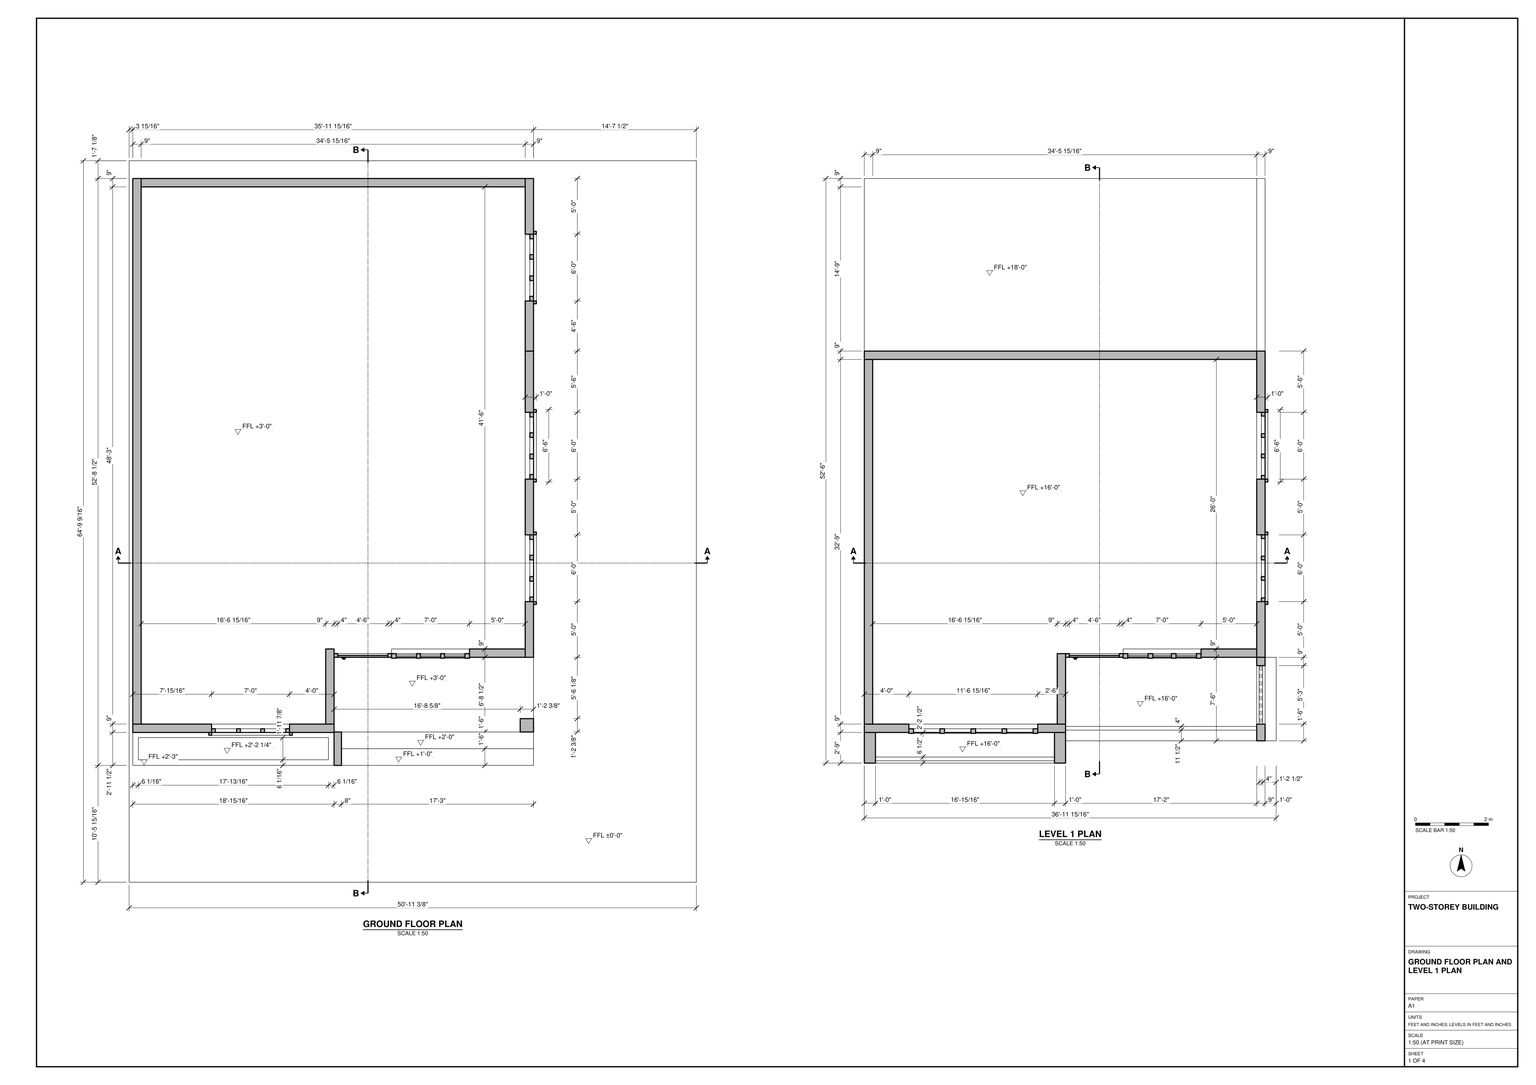
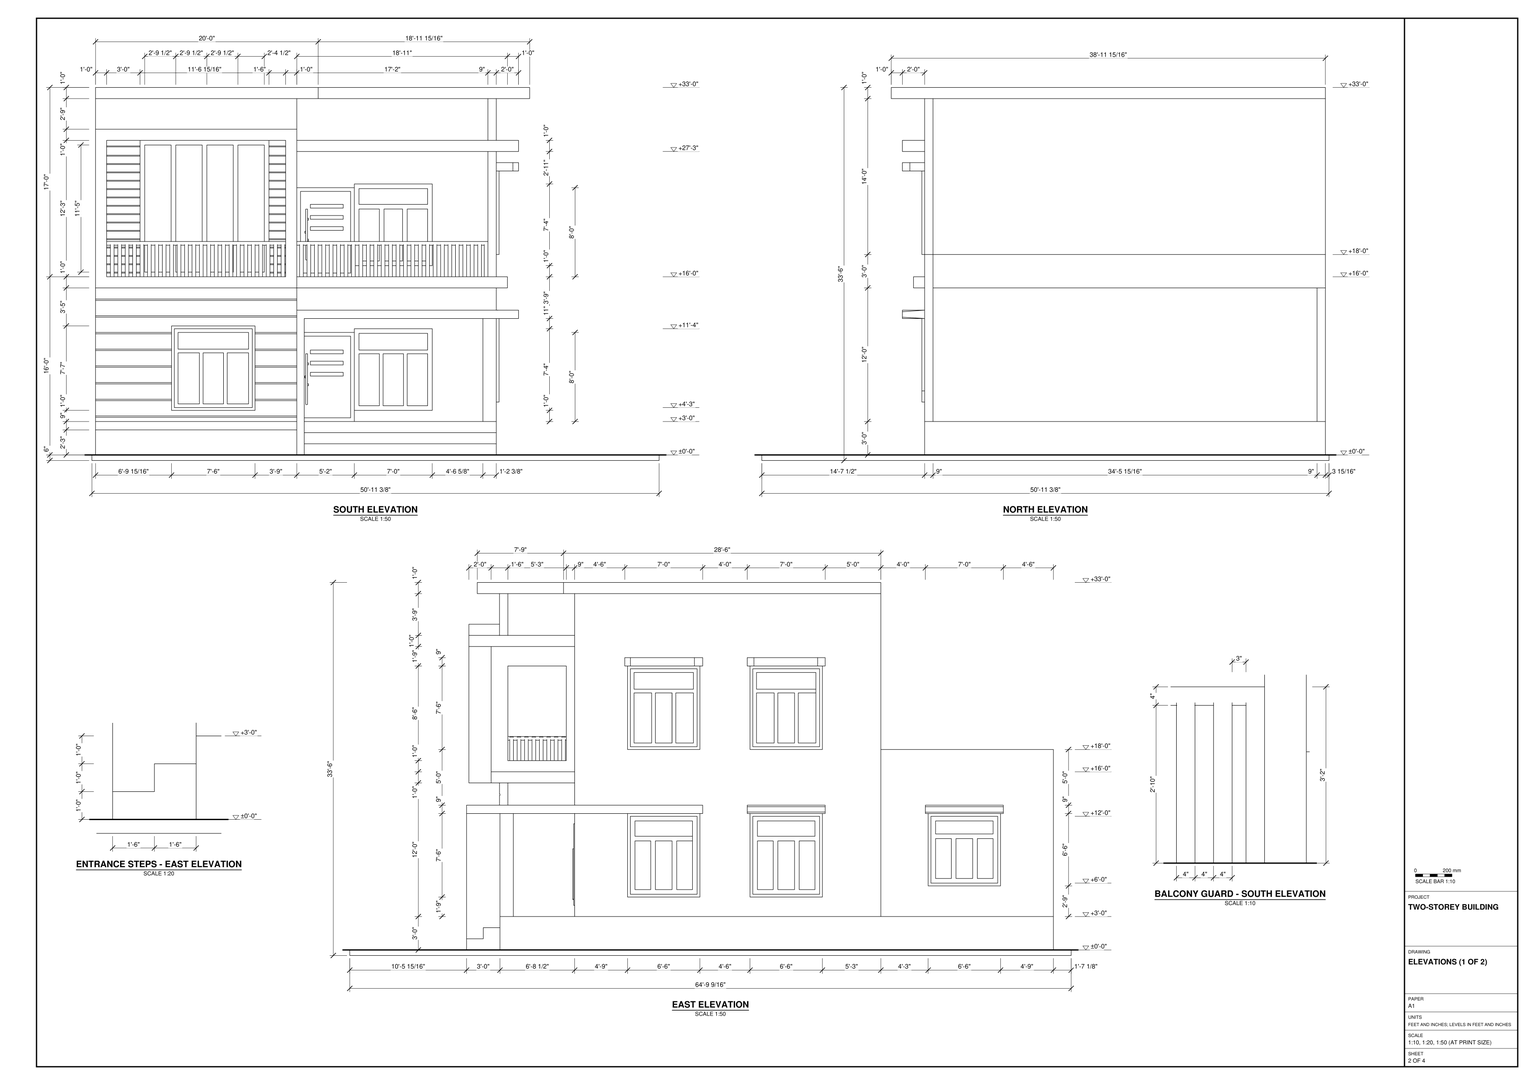
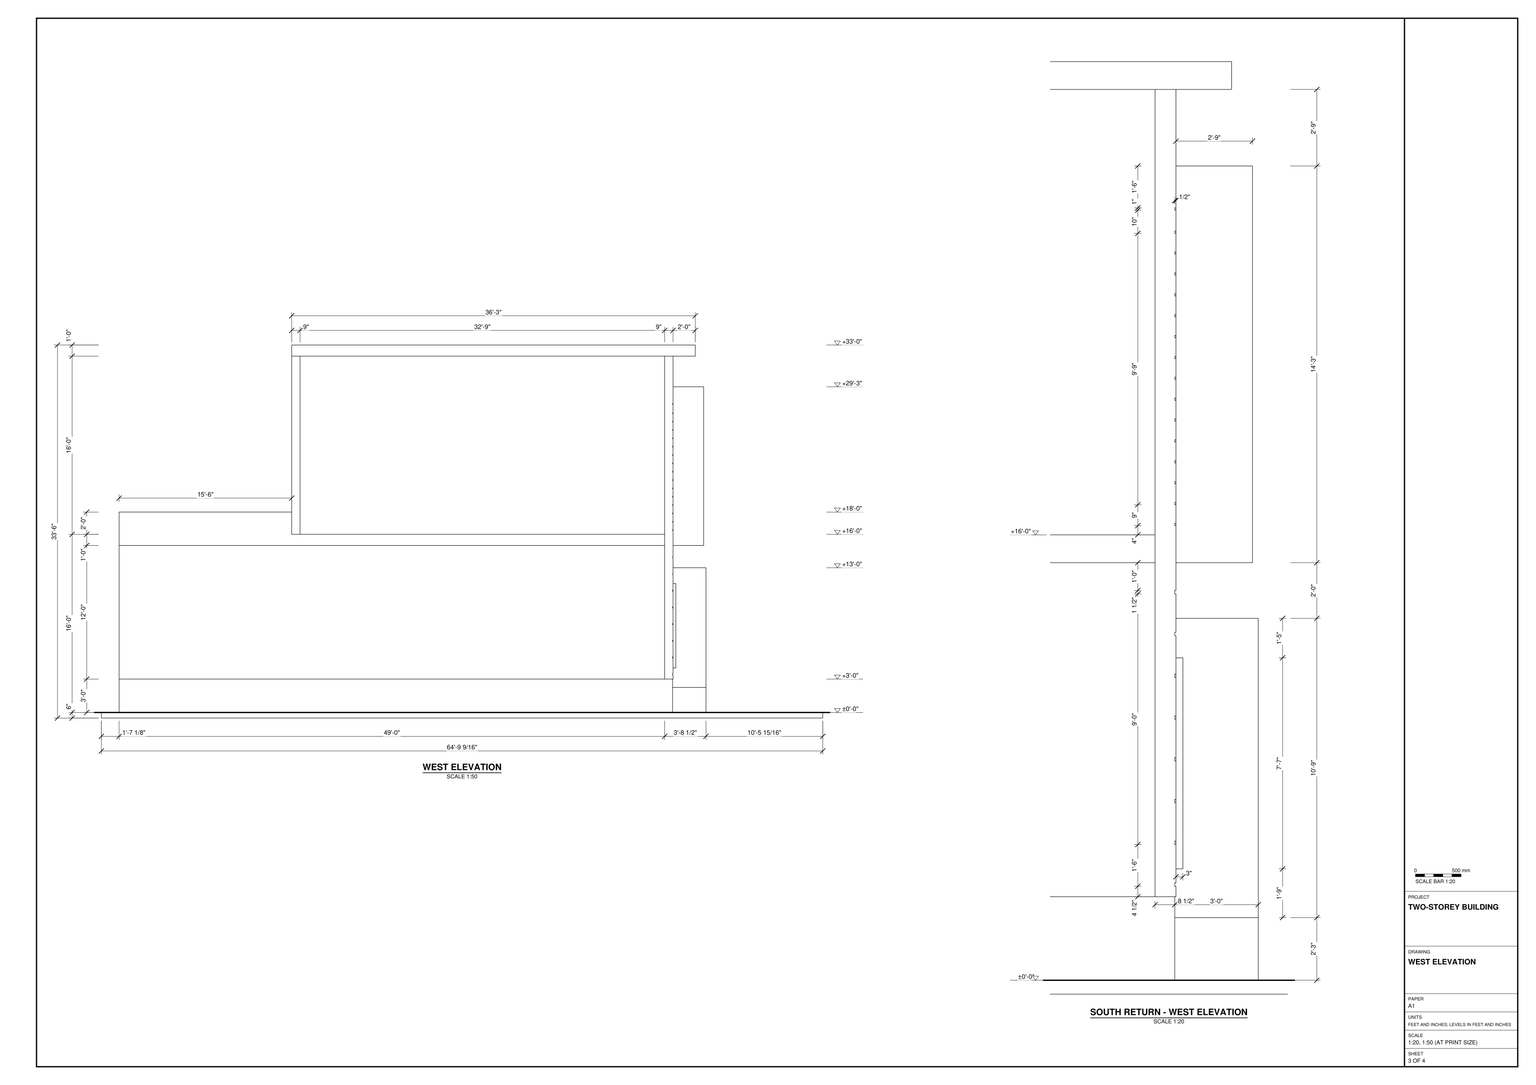
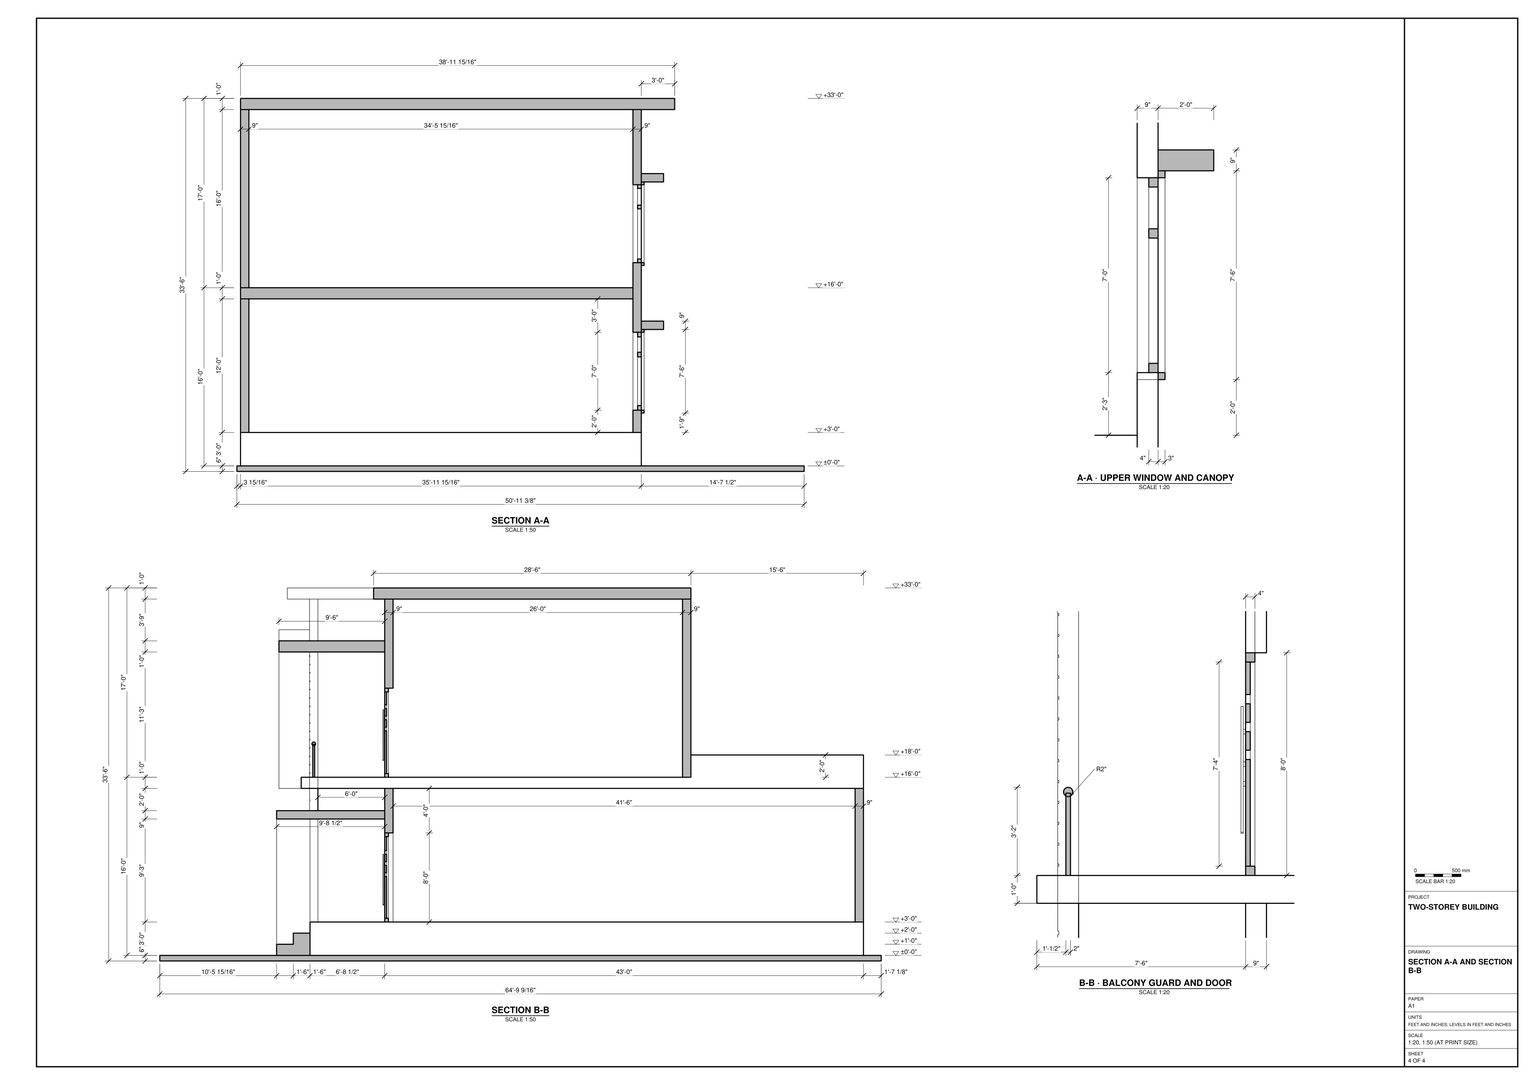
Build the two-storey building and its rectangular site base in SketchUp using task_files/diagram_01.pdf. Work in feet and inches. With north at the top of the plan, make the complete model 50'-11 3/8" wide, 64'-9 9/16" deep and 33'-6" high, including the base. Use ±0'-0" as the ground datum and +16'-0" as the upper storey level. Raise the ground floor and entrance landing to +3'-0" above the datum.

Set out the perimeter walls at the thicknesses drawn, retaining the recess at the south entrance. Model the floor slabs, the lower rear roof with its raised edge, and the flat overhanging roof above the shorter upper storey. Build the entrance steps, the porch supports and the upper balcony with its vertical guard bars. Use the south elevation to place the doors and divided windows, the horizontal bands on the projecting bay and the canopies over the recessed bay. Match the east window openings and their projecting heads to the elevation; keep the north and west walls unpierced.

Keep walls, slabs and roofs in separate groups or components. Group each furniture or joinery piece separately where shown, and use components for repeated parts. Any decor or loose items shown may be suitable library components. Save one SketchUp model as output_files/two_storey_building_with_stepped_entrance_and_balcony.skp.

# SketchUp Ruby script. Lengths in inches.
U = 1.inch
M = Sketchup.active_model
def pt(a) = Geom::Point3d.new(a.map { |v| v * U })
def face(e, loops, mat)
  f = e.add_face(loops[0].map { |a| pt(a) })
  loops[1..].each { |l| e.add_face(l.map { |a| pt(a) }).erase! }
  f.material = f.back_material = mat if mat
  f
end
# faces: each face lists its corners as indices into pts; further lists are holes
def faces(e, pts, list, mat = nil) = list.each { |f| face(e, (f[0].is_a?(Array) ? f : [f]).map { |l| l.map { |i| pts[i] } }, mat) }
# xy, xz, yz: faces in a plane at the given z, y or x. An outline is a flat list of corners, or four numbers for a rectangle; further outlines are holes
def ring(l) = l.size == 4 ? [[l[0], l[1]], [l[2], l[1]], [l[2], l[3]], [l[0], l[3]]] : l.each_slice(2).to_a
def flat(e, list, mat, &to3) = list.each { |f| face(e, (f[0].is_a?(Array) ? f : [f]).map { |l| ring(l).map { |u, v| to3.(u, v) } }, mat) }
def xy(e, z, list, mat = nil) = flat(e, list, mat) { |x, y| [x, y, z] }
def xz(e, y, list, mat = nil) = flat(e, list, mat) { |x, z| [x, y, z] }
def yz(e, x, list, mat = nil) = flat(e, list, mat) { |y, z| [x, y, z] }
def lines(e, pts, list) = list.each { |a, b| e.add_line(pt(pts[a]), pt(pts[b])) }
# prism: a flat outline (further loops are holes) pulled along v
def prism(e, loops, v, mat = nil)
  f = face(e, loops, mat); d = Geom::Vector3d.new(v.map { |x| x * U })
  f.pushpull(f.normal.samedirection?(d) ? d.length : -d.length)
end
def box(e, o, s, mat = nil) = prism(e, [[o, [o[0] + s[0], o[1], o[2]], [o[0] + s[0], o[1] + s[1], o[2]], [o[0], o[1] + s[1], o[2]]]], [0, 0, s[2]], mat)
def at(x, y, z, deg = 0) = Geom::Transformation.translation(pt([x, y, z])) * Geom::Transformation.rotation(ORIGIN, Z_AXIS, deg.degrees)
def axes(o, x, y, z) = Geom::Transformation.new([*x, 0, *y, 0, *z, 0, *pt(o).to_a, 1])
def part(name) = M.definitions.add(name)
# library, detail: a bought-in or finely detailed component or shape, given as its bounding box
def library(name, o, s) = part(name).tap { |d| box(d.entities, o, s) }
def detail(e, o, s) = box(e.add_group.entities, o, s)
def put(e, d, t, mat = nil) = e.add_instance(d, t).tap { |i| i.material = mat if mat }
def group(e, t, mat = nil) = e.add_group.tap { |g| g.transformation = t; g.material = mat if mat }.entities
root = M.entities
M.materials.add("[Color D06]").color = [142, 107, 0]
M.materials.add("[Color M02]").color = [198, 198, 198]
M.materials.add("[Color M04]").color = [142, 142, 142]
M.materials.add("[Color M05]").color = [114, 114, 114]
M.materials.add("[Color M06]").color = [86, 86, 86]
M.materials.add("[Color M09]").color = [0, 0, 0]
M.materials.add("[Grass Dark Green]").color = [106, 157, 55]
M.materials.add("[Pavers with Grass Brick]").color = [187, 192, 176]
M.materials.add("[Translucent Glass Gray]").color = [128, 128, 128]
M.materials["[Translucent Glass Gray]"].alpha = 0.5
M.materials.add("[Wood Veneer 01]").color = [109, 63, 33]
M.materials.add("[Wood Veneer 01]1").color = [73, 43, 22]
c1 = part("Group\#26")
box(c1.entities,[0,0,0],[3,1,2])
c2 = part("Group\#27")
box(c2.entities,[-1,0,0],[3,1,2])
c3 = part("Group\#28")
box(c3.entities,[0,0,0],[3,1,2])
c4 = part("Group\#29")
prism(c4.entities,[[[0,1,30.5],[2,1,30.5],[2,1,-23.76],[2,1,-23.82],[1.98,1,-23.88],[1.96,1,-23.94],[1.93,1,-24],[1.9,1,-24.06],[1.86,1,-24.11],[1.81,1,-24.15],[1.75,1,-24.18],[1.69,1,-24.21],[1.63,1,-24.23],[1.57,1,-24.25],[1.51,1,-24.25],[0.52,1,-24.25],[0.45,1,-24.25],[0.38,1,-24.23],[0.32,1,-24.21],[0.26,1,-24.18],[0.2,1,-24.14],[0.15,1,-24.1],[0.11,1,-24.05],[0.07,1,-23.99],[0.04,1,-23.93],[0.02,1,-23.87],[0,1,-23.8],[0,1,-23.73]]],[0,-1,0])
c5 = part("Group\#40")
prism(c5.entities,[[[74,0.51,0.02],[74,0.6875,0],[74,0.87,0.02],[74,1.03,0.09],[74,1.17,0.2],[74,1.28,0.34],[74,1.35,0.51],[74,1.375,0.6875],[74,1.35,0.87],[74,1.28,1.03],[74,1.17,1.17],[74,1.03,1.28],[74,0.87,1.35],[74,0.6875,1.375],[74,0.51,1.35],[74,0.34,1.28],[74,0.2,1.17],[74,0.09,1.03],[74,0.02,0.87],[74,0,0.6875],[74,0.02,0.51],[74,0.09,0.34],[74,0.2,0.2],[74,0.34,0.09]]],[-74,0,0])
c6 = part("Group\#31")
prism(c6.entities,[[[1.4,0.375,0],[1.28,0.22,0],[1.125,0.1,0],[0.94,0.03,0],[0.75,0,0],[0.56,0.03,0],[0.375,0.1,0],[0.22,0.22,0],[0.1,0.375,0],[0.03,0.56,0],[0,0.75,0],[0.03,0.94,0],[0.1,1.125,0],[0.22,1.28,0],[0.375,1.4,0],[0.56,1.47,0],[0.75,1.5,0],[0.94,1.47,0],[1.125,1.4,0],[1.28,1.28,0],[1.4,1.125,0],[1.47,0.94,0],[1.5,0.75,0],[1.47,0.56,0]]],[0,0,18])
c7 = part("Group\#60")
prism(c7.entities,[[[0,0.16,0.96],[0,0.28,1.05],[0,0.42,1.11],[0,0.5625,1.125],[0,0.71,1.11],[0,0.84,1.05],[0,0.96,0.96],[0,1.05,0.84],[0,1.11,0.71],[0,1.125,0.5625],[0,1.11,0.42],[0,1.05,0.28],[0,0.96,0.16],[0,0.84,0.08],[0,0.71,0.02],[0,0.5625,0],[0,0.42,0.02],[0,0.28,0.08],[0,0.16,0.16],[0,0.08,0.28],[0,0.02,0.42],[0,0,0.5625],[0,0.02,0.71],[0,0.08,0.84]]],[74,0,0])
c8 = part("Group\#61")
prism(c8.entities,[[[1.25,0.625,0],[1.23,0.46,0],[1.17,0.3125,0],[1.07,0.18,0],[0.9375,0.08,0],[0.79,0.02,0],[0.625,0,0],[0.46,0.02,0],[0.3125,0.08,0],[0.18,0.18,0],[0.08,0.3125,0],[0.02,0.46,0],[0,0.625,0],[0.02,0.79,0],[0.08,0.9375,0],[0.18,1.07,0],[0.3125,1.17,0],[0.46,1.23,0],[0.625,1.25,0],[0.79,1.23,0],[0.9375,1.17,0],[1.07,1.07,0],[1.17,0.9375,0],[1.23,0.79,0]]],[0,0,17])
c9 = part("Group\#87")
box(c9.entities,[0,0,0],[4,2,35.48])
c10 = part("Group\#85")
box(c10.entities,[0,0,0],[4,2,25.41])
g1 = group(root,at(0,153.25,0))
xy(g1,0,[[0,-153.25,611.36,624.3125]])
xy(g1,6,[[0,-153.25,611.36,624.3125]],"[Pavers with Grass Brick]")
xz(g1,-153.25,[[0,0,611.36,6]])
xz(g1,624.3125,[[0,0,611.36,6]])
yz(g1,0,[[-153.25,0,624.3125,6]])
yz(g1,611.36,[[-153.25,0,624.3125,6]])
g2 = group(root,at(75.86,338.41,6),"[Color M02]")
box(g2,[-71.9375,-176.5,0],[431.9375,596.5,36])
g3 = group(root,at(75.86,242.41,42),"[Color M02]")
xy(g3,0,[[207,0,351,9]])
xy(g3,12,[[207,0,291,9]])
xy(g3,96,[[145,0,207,9]])
xy(g3,100,[[207,0,291,9]])
xy(g3,144,[[145,0,351,9]])
xz(g3,0,[[207,0,351,0,351,144,145,144,145,96,207,96,207,100,291,100,291,12,207,12]])
xz(g3,9,[[207,0,207,12,291,12,291,100,207,100,207,96,145,96,145,144,351,144,351,0]])
yz(g3,145,[[0,0,9,96],[0,96,9,144]])
yz(g3,207,[[0,0,9,12],[0,96,9,100]])
yz(g3,291,[[0,12,9,100]])
yz(g3,351,[[0,0,9,144]])
g4 = group(root,at(431.86,302.41,66),"[Color M09]")
xy(g4,0,[[0,0,4,72]])
xy(g4,5,[[0,5,4,22],[0,27,4,45],[0,50,4,67]])
xy(g4,57.5,[[0,5,4,22],[0,27,4,45],[0,50,4,67]])
xy(g4,62.5,[[0,5,4,67]])
xy(g4,79,[[0,5,4,67]])
xy(g4,84,[[0,0,4,72]])
xz(g4,0,[[0,0,4,84]])
xz(g4,5,[[0,5,4,57.5],[0,62.5,4,79]])
xz(g4,22,[[0,5,4,57.5]])
xz(g4,27,[[0,5,4,57.5]])
xz(g4,45,[[0,5,4,57.5]])
xz(g4,50,[[0,5,4,57.5]])
xz(g4,67,[[0,5,4,57.5],[0,57.5,4,62.5],[0,62.5,4,79]])
xz(g4,72,[[0,0,4,84]])
yz(g4,0,[[[0,0,72,84],[50,5,67,5,67,79,5,79,5,62.5,67,62.5,67,57.5,50,57.5],[27,5,45,57.5],[5,5,22,57.5]]])
yz(g4,4,[[[0,0,72,84],[50,5,50,57.5,67,57.5,67,62.5,5,62.5,5,79,67,79,67,5],[27,5,45,57.5],[5,5,22,57.5]]])
g5 = group(root,at(435.86,299.41,63),"[Color M06]")
prism(g5,[[[0,0,0],[0,0,90],[0,78,90],[0,78,0]],[[0,3,87],[0,3,3],[0,75,3],[0,75,87]]],[3,0,0])
g6 = group(root,at(435.86,307.41,128.5),"[Translucent Glass Gray]")
yz(g6,0,[[0,0,62,16.5]])
g7 = group(root,at(435.86,352.41,71),"[Translucent Glass Gray]")
yz(g7,0,[[0,0,17,52.5]])
g8 = group(root,at(435.86,329.41,71),"[Translucent Glass Gray]")
yz(g8,0,[[0,0,18,52.5]])
g9 = group(root,at(435.86,307.41,71),"[Translucent Glass Gray]")
yz(g9,0,[[0,0,17,52.5]])
g10 = group(root,at(431.86,434.41,66),"[Color M09]")
prism(g10,[[[0,72,84],[0,72,0],[0,0,0],[0,0,84]],[[0,67,62.5],[0,67,79],[0,5,79],[0,5,62.5]],[[0,45,5],[0,45,57.5],[0,27,57.5],[0,27,12],[0,27,5]],[[0,22,5],[0,22,57.5],[0,5,57.5],[0,5,5]],[[0,67,57.5],[0,50,57.5],[0,50,5],[0,67,5]]],[4,0,0])
g11 = group(root,at(435.86,431.41,63),"[Color M06]")
prism(g11,[[[0,78,90],[0,78,0],[0,0,0],[0,0,90]],[[0,75,3],[0,75,87],[0,3,87],[0,3,3]]],[3,0,0])
g12 = group(root,at(431.86,626.41,78),"[Color M09]")
prism(g12,[[[0,0,0],[0,0,72],[0,72,72],[0,72,0]],[[0,67,53],[0,67,67],[0,5,67],[0,5,53]],[[0,45,5],[0,45,48],[0,27,48],[0,27,5]],[[0,67,48],[0,50,48],[0,50,5],[0,67,5]],[[0,5,48],[0,5,5],[0,22,5],[0,22,48]]],[4,0,0])
g13 = group(root,at(435.86,623.41,75),"[Color M06]")
prism(g13,[[[0,0,78],[0,78,78],[0,78,0],[0,0,0]],[[0,75,75],[0,3,75],[0,3,3],[0,75,3]]],[3,0,0])
g14 = group(root,at(435.86,439.41,128.5),"[Translucent Glass Gray]")
yz(g14,0,[[0,0,62,16.5]])
g15 = group(root,at(435.86,439.41,71),"[Translucent Glass Gray]")
yz(g15,0,[[0,0,17,52.5]])
g16 = group(root,at(435.86,461.41,71),"[Translucent Glass Gray]")
yz(g16,0,[[0,0,18,52.5]])
g17 = group(root,at(435.86,484.41,71),"[Translucent Glass Gray]")
yz(g17,0,[[0,0,17,52.5]])
g18 = group(root,at(435.86,631.41,131),"[Translucent Glass Gray]")
yz(g18,0,[[0,0,62,14]])
g19 = group(root,at(435.86,676.41,83),"[Translucent Glass Gray]")
yz(g19,0,[[0,0,17,43]])
g20 = group(root,at(435.86,653.41,83),"[Translucent Glass Gray]")
yz(g20,0,[[0,0,18,43]])
g21 = group(root,at(435.86,631.41,83),"[Translucent Glass Gray]")
yz(g21,0,[[0,0,17,43]])
g22 = group(root,at(282.86,242.41,42),"[Wood Veneer 01]")
prism(g22,[[[0,4,12],[0,4,100],[84,4,100],[84,4,12]],[[5,4,77],[79,4,77],[79,4,95],[5,4,95]],[[57,4,73],[57,4,17],[79,4,17],[79,4,73]],[[5,4,17],[27,4,17],[27,4,73],[5,4,73]],[[31,4,17],[53,4,17],[53,4,73],[31,4,73]]],[0,-5,0])
g23 = group(root,at(220.86,242.41,42),"[Wood Veneer 01]")
prism(g23,[[[62,4,0],[0,4,0],[0,4,96],[62,4,96]],[[58,4,92],[4,4,92],[4,4,4],[58,4,4]]],[0,-4,0])
g24 = group(root,at(224.86,242.41,46),"[Wood Veneer 01]")
prism(g24,[[[0,2,0],[0,2,88],[54,2,88],[54,2,0]],[[10.6,2,73],[10.6,2,69],[46,2,69],[46,2,73]],[[10.6,2,57],[46,2,57],[46,2,61],[10.6,2,61]],[[10.6,2,49],[10.6,2,45],[46,2,45],[46,2,49]]],[0,-2,0])
put(root,c1,at(230.46,241.41,103.125))
put(root,c2,at(230.46,241.41,89.1))
put(root,c3,at(230.46,241.41,80.625))
put(root,c4,at(230.46,240.41,84.5))
put(root,c5,at(287.86,243.72,110.26))
put(root,c5,at(287.86,243.72,104.26))
put(root,c5,at(287.86,243.72,98.26))
put(root,c5,at(287.86,243.72,92.26))
put(root,c5,at(287.86,243.72,86.26))
put(root,c5,at(287.86,243.72,80.26))
put(root,c5,at(287.86,243.72,74.26))
put(root,c5,at(287.86,243.72,68.26))
put(root,c5,at(287.86,243.72,62.26))
put(root,c6,at(288.87,243.66,119))
put(root,c6,at(293.87,243.66,119))
put(root,c6,at(298.87,243.66,119))
put(root,c6,at(303.87,243.66,119))
put(root,c6,at(308.87,243.66,119))
put(root,c6,at(313.87,243.66,119))
put(root,c6,at(318.87,243.66,119))
put(root,c6,at(323.87,243.66,119))
put(root,c6,at(328.87,243.66,119))
put(root,c6,at(333.87,243.66,119))
put(root,c6,at(338.87,243.66,119))
put(root,c6,at(343.87,243.66,119))
put(root,c6,at(348.87,243.66,119))
put(root,c6,at(353.87,243.66,119))
put(root,c6,at(358.87,243.66,119))
g25 = group(root,at(235.46,242.41,115),"[Translucent Glass Gray]")
xz(g25,0,[[0,0,35.4,4]])
g26 = group(root,at(235.46,242.41,103),"[Translucent Glass Gray]")
xz(g26,0,[[0,0,35.4,4]])
g27 = group(root,at(235.46,242.41,91),"[Translucent Glass Gray]")
xz(g27,0,[[0,0,35.4,4]])
g28 = group(root,at(287.86,242.41,119),"[Translucent Glass Gray]")
xz(g28,0,[[0,0,74,18]])
g29 = group(root,at(287.86,242.41,59),"[Translucent Glass Gray]")
xz(g29,0,[[0,0,22,56]])
g30 = group(root,at(313.86,242.41,59),"[Translucent Glass Gray]")
xz(g30,0,[[0,0,22,56]])
g31 = group(root,at(339.86,242.41,59),"[Translucent Glass Gray]")
xz(g31,0,[[0,0,22,56]])
g32 = group(root,at(211.86,170.41,42))
box(g32,[0,0,0],[9,81,144])
g33 = group(root,at(75.86,161.41,42),"[Color M02]")
xy(g33,0,[[-71.9375,0,145,9]])
xy(g33,4.5,[[-71.9375,0,145,0.5]])
xy(g33,6,[[-71.9375,0,145,0.5]])
xy(g33,15,[[13,0,97,9]])
xy(g33,22.5,[[-71.9375,0,13,0.5],[97,0,145,0.5]])
xy(g33,24,[[-71.9375,0,13,0.5],[97,0,145,0.5]])
xy(g33,40.5,[[-71.9375,0,13,0.5],[97,0,145,0.5]])
xy(g33,42,[[-71.9375,0,13,0.5],[97,0,145,0.5]])
xy(g33,58.5,[[-71.9375,0,13,0.5],[97,0,145,0.5]])
xy(g33,60,[[-71.9375,0,13,0.5],[97,0,145,0.5]])
xy(g33,76.5,[[-71.9375,0,13,0.5],[97,0,145,0.5]])
xy(g33,78,[[-71.9375,0,13,0.5],[97,0,145,0.5]])
xy(g33,94.5,[[-71.9375,0,13,0.5],[97,0,145,0.5]])
xy(g33,96,[[-71.9375,0,13,0.5],[97,0,145,0.5]])
xy(g33,100,[[13,0,97,9]])
xy(g33,112.5,[[-71.9375,0,145,0.5]])
xy(g33,114,[[-71.9375,0,145,0.5]])
xy(g33,130.5,[[-71.9375,0,145,0.5]])
xy(g33,132,[[-71.9375,0,145,0.5]])
xy(g33,156,[[-23.9375,0,115,9]])
xy(g33,159.97,[[-71.9375,0,-23.9375,0.5],[115,0,145,0.5]])
xy(g33,160.97,[[-71.9375,0,-23.9375,0.5],[115,0,145,0.5]])
xy(g33,168.97,[[-71.9375,0,-23.9375,0.5],[115,0,145,0.5]])
xy(g33,169.97,[[-71.9375,0,-23.9375,0.5],[115,0,145,0.5]])
xy(g33,177.97,[[-71.9375,0,-23.9375,0.5],[115,0,145,0.5]])
xy(g33,178.97,[[-71.9375,0,-23.9375,0.5],[115,0,145,0.5]])
xy(g33,186.97,[[-71.9375,0,-23.9375,0.5],[115,0,145,0.5]])
xy(g33,187.97,[[-71.9375,0,-23.9375,0.5],[115,0,145,0.5]])
xy(g33,195.97,[[-71.9375,0,-23.9375,0.5],[115,0,145,0.5]])
xy(g33,196.97,[[-71.9375,0,-23.9375,0.5],[115,0,145,0.5]])
xy(g33,204.97,[[-71.9375,0,-23.9375,0.5],[115,0,145,0.5]])
xy(g33,205.97,[[-71.9375,0,-23.9375,0.5],[115,0,145,0.5]])
xy(g33,213.97,[[-71.9375,0,-23.9375,0.5],[115,0,145,0.5]])
xy(g33,214.97,[[-71.9375,0,-23.9375,0.5],[115,0,145,0.5]])
xy(g33,222.97,[[-71.9375,0,-23.9375,0.5],[115,0,145,0.5]])
xy(g33,223.97,[[-71.9375,0,-23.9375,0.5],[115,0,145,0.5]])
xy(g33,231.97,[[-71.9375,0,-23.9375,0.5],[115,0,145,0.5]])
xy(g33,232.97,[[-71.9375,0,-23.9375,0.5],[115,0,145,0.5]])
xy(g33,240.97,[[-71.9375,0,-23.9375,0.5],[115,0,145,0.5]])
xy(g33,241.97,[[-71.9375,0,-23.9375,0.5],[115,0,145,0.5]])
xy(g33,249.97,[[-71.9375,0,-23.9375,0.5],[115,0,145,0.5]])
xy(g33,250.97,[[-71.9375,0,-23.9375,0.5],[115,0,145,0.5]])
xy(g33,258.97,[[-71.9375,0,-23.9375,0.5],[115,0,145,0.5]])
xy(g33,259.97,[[-71.9375,0,-23.9375,0.5],[115,0,145,0.5]])
xy(g33,267.97,[[-71.9375,0,-23.9375,0.5],[115,0,145,0.5]])
xy(g33,268.97,[[-71.9375,0,-23.9375,0.5],[115,0,145,0.5]])
xy(g33,276.97,[[-71.9375,0,-23.9375,0.5],[115,0,145,0.5]])
xy(g33,277.97,[[-71.9375,0,-23.9375,0.5],[115,0,145,0.5]])
xy(g33,285.97,[[-71.9375,0,-23.9375,0.5],[115,0,145,0.5]])
xy(g33,286.97,[[-71.9375,0,-23.9375,0.5],[115,0,145,0.5]])
xy(g33,295.97,[[-71.9375,0,-23.9375,0.5],[115,0,145,0.5]])
xy(g33,296.97,[[-71.9375,0,-23.9375,0.5],[115,0,145,0.5]])
xy(g33,303,[[-23.9375,0,115,9]])
xy(g33,348,[[-71.9375,0,145,9]])
xz(g33,0,[[-71.9375,0,145,4.5],[-71.9375,6,145,6,145,22.5,97,22.5,97,15,13,15,13,22.5,-71.9375,22.5],[-71.9375,24,13,40.5],[97,24,145,40.5],[-71.9375,42,13,58.5],
  [97,42,145,58.5],[-71.9375,60,13,76.5],[97,60,145,76.5],[-71.9375,78,13,94.5],[97,78,145,94.5],
  [-71.9375,96,13,96,13,100,97,100,97,96,145,96,145,112.5,-71.9375,112.5],[-71.9375,114,145,130.5],[-71.9375,132,145,132,145,159.97,115,159.97,115,156,-23.9375,156,-23.9375,159.97,-71.9375,159.97],[-71.9375,315,145,348]])
xz(g33,0,[[-71.9375,160.97,-23.9375,168.97],[115,160.97,145,168.97],[-71.9375,169.97,-23.9375,177.97],[115,169.97,145,177.97],[-71.9375,178.97,-23.9375,186.97],
  [115,178.97,145,186.97],[-71.9375,187.97,-23.9375,195.97],[115,187.97,145,195.97],[-71.9375,196.97,-23.9375,204.97],[115,196.97,145,204.97],
  [-71.9375,205.97,-23.9375,213.97],[115,205.97,145,213.97],[-71.9375,214.97,-23.9375,222.97],[115,214.97,145,222.97],[-71.9375,223.97,-23.9375,231.97],
  [115,223.97,145,231.97],[-71.9375,232.97,-23.9375,240.97],[115,232.97,145,240.97],[-71.9375,241.97,-23.9375,249.97],[115,241.97,145,249.97],
  [-71.9375,250.97,-23.9375,258.97],[115,250.97,145,258.97],[-71.9375,259.97,-23.9375,267.97],[115,259.97,145,267.97],[-71.9375,268.97,-23.9375,276.97],
  [115,268.97,145,276.97],[-71.9375,277.97,-23.9375,285.97],[115,277.97,145,285.97],[-71.9375,286.97,-23.9375,295.97],[115,286.97,145,295.97],
  [-71.9375,296.97,-23.9375,296.97,-23.9375,303,115,303,115,296.97,145,296.97,145,315,-71.9375,315]],"[Color D06]")
xz(g33,0.5,[[-71.9375,4.5,145,6],[-71.9375,22.5,13,24],[97,22.5,145,24],[-71.9375,40.5,13,42],[97,40.5,145,42],
  [-71.9375,58.5,13,60],[97,58.5,145,60],[-71.9375,76.5,13,78],[97,76.5,145,78],[-71.9375,94.5,13,96],
  [97,94.5,145,96],[-71.9375,112.5,145,114],[-71.9375,130.5,145,132]],"[Color M05]")
xz(g33,0.5,[[-71.9375,159.97,-23.9375,160.97],[115,159.97,145,160.97],[-71.9375,168.97,-23.9375,169.97],[115,168.97,145,169.97],[-71.9375,177.97,-23.9375,178.97],
  [115,177.97,145,178.97],[-71.9375,186.97,-23.9375,187.97],[115,186.97,145,187.97],[-71.9375,195.97,-23.9375,196.97],[115,195.97,145,196.97],
  [-71.9375,204.97,-23.9375,205.97],[115,204.97,145,205.97],[-71.9375,213.97,-23.9375,214.97],[115,213.97,145,214.97],[-71.9375,222.97,-23.9375,223.97],
  [115,222.97,145,223.97],[-71.9375,231.97,-23.9375,232.97],[115,231.97,145,232.97],[-71.9375,240.97,-23.9375,241.97],[115,240.97,145,241.97],
  [-71.9375,249.97,-23.9375,250.97],[115,249.97,145,250.97],[-71.9375,258.97,-23.9375,259.97],[115,258.97,145,259.97],[-71.9375,267.97,-23.9375,268.97],
  [115,267.97,145,268.97],[-71.9375,276.97,-23.9375,277.97],[115,276.97,145,277.97],[-71.9375,285.97,-23.9375,286.97],[115,285.97,145,286.97],
  [-71.9375,295.97,-23.9375,296.97],[115,295.97,145,296.97]],"[Color M09]")
xz(g33,9,[[[-71.9375,0,145,348],[-23.9375,156,115,303],[13,15,97,100]]])
yz(g33,-71.9375,[[0,0,0,4.5,0.5,4.5,0.5,6,0,6,0,22.5,0.5,22.5,0.5,24,0,24,0,40.5,0.5,40.5,0.5,42,0,42,0,58.5,0.5,58.5,0.5,60,0,60,0,76.5,0.5,76.5,0.5,78,0,78,0,94.5,0.5,94.5,0.5,96,0,96,0,112.5,0.5,112.5,0.5,114,0,114,0,130.5,0.5,130.5,0.5,132,0,132,0,159.97,0.5,159.97,0.5,160.97,0,160.97,0,168.97,0.5,168.97,0.5,169.97,0,169.97,0,177.97,0.5,177.97,0.5,178.97,0,178.97,0,186.97,0.5,186.97,0.5,187.97,0,187.97,0,195.97,0.5,195.97,0.5,196.97,0,196.97,0,204.97,0.5,204.97,0.5,205.97,0,205.97,0,213.97,0.5,213.97,0.5,214.97,0,214.97,0,222.97,0.5,222.97,0.5,223.97,0,223.97,0,231.97,0.5,231.97,0.5,232.97,0,232.97,0,240.97,0.5,240.97,0.5,241.97,0,241.97,0,249.97,0.5,249.97,0.5,250.97,0,250.97,0,258.97,0.5,258.97,0.5,259.97,0,259.97,0,267.97,0.5,267.97,0.5,268.97,0,268.97,0,276.97,0.5,276.97,0.5,277.97,0,277.97,0,285.97,0.5,285.97,0.5,286.97,0,286.97,0,295.97,0.5,295.97,0.5,296.97,0,296.97,0,348,9,348,9,0]])
yz(g33,-23.9375,[[0,156,9,156,9,303,0.5,303,0.5,285.97,0,285.97,0,277.97,0.5,277.97,0.5,276.97,0,276.97,0,268.97,0.5,268.97,0.5,267.97,0,267.97,0,259.97,0.5,259.97,0.5,258.97,0,258.97,0,250.97,0.5,250.97,0.5,249.97,0,249.97,0,241.97,0.5,241.97,0.5,240.97,0,240.97,0,232.97,0.5,232.97,0.5,231.97,0,231.97,0,223.97,0.5,223.97,0.5,222.97,0,222.97,0,214.97,0.5,214.97,0.5,213.97,0,213.97,0,205.97,0.5,205.97,0.5,204.97,0,204.97,0,196.97,0.5,196.97,0.5,195.97,0,195.97,0,187.97,0.5,187.97,0.5,186.97,0,186.97,0,178.97,0.5,178.97,0.5,177.97,0,177.97,0,169.97,0.5,169.97,0.5,168.97,0,168.97,0,160.97,0.5,160.97,0.5,159.97,0,159.97],[0,286.97,0.5,295.97],[0,296.97,0.5,303]])
yz(g33,13,[[0,15,9,15,9,100,0,100,0,96,0.5,96,0.5,94.5,0,94.5,0,78,0.5,78,0.5,76.5,0,76.5,0,60,0.5,60,0.5,58.5,0,58.5,0,42,0.5,42,0.5,40.5,0,40.5,0,24,0.5,24,0.5,22.5,0,22.5]])
yz(g33,97,[[0,15,0,22.5,0.5,22.5,0.5,24,0,24,0,40.5,0.5,40.5,0.5,42,0,42,0,58.5,0.5,58.5,0.5,60,0,60,0,76.5,0.5,76.5,0.5,78,0,78,0,94.5,0.5,94.5,0.5,96,0,96,0,100,9,100,9,15]])
yz(g33,115,[[0,156,0,159.97,0.5,159.97,0.5,160.97,0,160.97,0,168.97,0.5,168.97,0.5,169.97,0,169.97,0,177.97,0.5,177.97,0.5,178.97,0,178.97,0,186.97,0.5,186.97,0.5,187.97,0,187.97,0,195.97,0.5,195.97,0.5,196.97,0,196.97,0,204.97,0.5,204.97,0.5,205.97,0,205.97,0,213.97,0.5,213.97,0.5,214.97,0,214.97,0,222.97,0.5,222.97,0.5,223.97,0,223.97,0,231.97,0.5,231.97,0.5,232.97,0,232.97,0,240.97,0.5,240.97,0.5,241.97,0,241.97,0,249.97,0.5,249.97,0.5,250.97,0,250.97,0,258.97,0.5,258.97,0.5,259.97,0,259.97,0,267.97,0.5,267.97,0.5,268.97,0,268.97,0,276.97,0.5,276.97,0.5,277.97,0,277.97,0,285.97,0.5,285.97,0.5,286.97,0,286.97,0,295.97,0.5,295.97,0.5,296.97,0,296.97,0,303,9,303,9,156]])
yz(g33,145,[[0,0,9,0,9,348,0,348,0,296.97,0.5,296.97,0.5,295.97,0,295.97,0,286.97,0.5,286.97,0.5,285.97,0,285.97,0,277.97,0.5,277.97,0.5,276.97,0,276.97,0,268.97,0.5,268.97,0.5,267.97,0,267.97,0,259.97,0.5,259.97,0.5,258.97,0,258.97,0,250.97,0.5,250.97,0.5,249.97,0,249.97,0,241.97,0.5,241.97,0.5,240.97,0,240.97,0,232.97,0.5,232.97,0.5,231.97,0,231.97,0,223.97,0.5,223.97,0.5,222.97,0,222.97,0,214.97,0.5,214.97,0.5,213.97,0,213.97,0,205.97,0.5,205.97,0.5,204.97,0,204.97,0,196.97,0.5,196.97,0.5,195.97,0,195.97,0,187.97,0.5,187.97,0.5,186.97,0,186.97,0,178.97,0.5,178.97,0.5,177.97,0,177.97,0,169.97,0.5,169.97,0.5,168.97,0,168.97,0,160.97,0.5,160.97,0.5,159.97,0,159.97,0,132,0.5,132,0.5,130.5,0,130.5,0,114,0.5,114,0.5,112.5,0,112.5,0,96,0.5,96,0.5,94.5,0,94.5,0,78,0.5,78,0.5,76.5,0,76.5,0,60,0.5,60,0.5,58.5,0,58.5,0,42,0.5,42,0.5,40.5,0,40.5,0,24,0.5,24,0.5,22.5,0,22.5,0,6,0.5,6,0.5,4.5,0,4.5]])
p = [[-59.9375,0,303],[-23.9375,-1,303],[-23.9375,-1,296.97],[-59.9375,0,296.97]]
lines(g33,p,[[0,1],[1,2],[0,3]])
g34 = group(root,at(85.86,158.41,54),"[Color M06]")
prism(g34,[[[90,3,91],[90,3,0],[0,3,0],[0,3,91]],[[3,3,88],[3,3,3],[87,3,3],[87,3,88]]],[0,-3,0])
g35 = group(root,at(88.86,161.41,57),"[Color M09]")
prism(g35,[[[0,4,0],[0,4,85],[84,4,85],[84,4,0]],[[4,4,63],[80,4,63],[80,4,81],[4,4,81]],[[27,4,4],[27,4,59],[4,4,59],[4,4,4]],[[80,4,59],[57,4,59],[57,4,4],[80,4,4]],[[53,4,4],[53,4,59],[31,4,59],[31,4,4]]],[0,-4,0])
g36 = group(root,at(145.86,161.41,61),"[Translucent Glass Gray]")
xz(g36,0,[[0,0,23,55]])
g37 = group(root,at(119.86,161.41,61),"[Translucent Glass Gray]")
xz(g37,0,[[0,0,22,55]])
g38 = group(root,at(92.86,161.41,61),"[Translucent Glass Gray]")
xz(g38,0,[[0,0,23,55]])
g39 = group(root,at(92.86,161.41,120),"[Translucent Glass Gray]")
xz(g39,0,[[0,0,76,18]])
g40 = group(root,at(220.86,170.41,162),"[Color M04]")
box(g40,[0,0,0],[215,72,24])
g41 = group(root,at(220.86,143.41,6),"[Color M02]")
xy(g41,0,[[0,-17.5,8,18.5]])
xy(g41,147,[[8,-17.5,8,18.5,0,18.5,0,99,215,99,215,237,239,237,239,-17.5]])
xy(g41,156,[[0,-17.5,239,-17.5,239,237,215,237,215,99,0,99]])
xz(g41,-17.5,[[0,0,8,0,8,147,239,147,239,156,0,156]])
xz(g41,18.5,[[0,0,8,147]])
xz(g41,99,[[0,147,215,156]])
xz(g41,237,[[215,147,239,156]])
yz(g41,0,[[-17.5,0,-17.5,156,99,156,99,147,18.5,147,18.5,0]])
yz(g41,8,[[-17.5,0,18.5,147]])
yz(g41,215,[[99,147,237,156]])
yz(g41,239,[[-17.5,147,237,156]])
p = [[0,18.5,148.5],[12,18.5,148]]
lines(g41,p,[[0,1]])
g42 = group(root,at(3.92,170.41,42),"[Color M02]")
box(g42,[0,0,0],[9,588,144])
g43 = group(root,at(3.92,170.41,186),"[Color M06]")
xy(g43,0,[[216.9375,-18,216.9375,0,0,0,0,588,422.9375,588,422.9375,72,443.9375,72,443.9375,-18]])
xy(g43,12,[[216.9375,-18,443.9375,-18,443.9375,72,422.9375,72,422.9375,402,0,402,0,0,216.9375,0]])
xy(g43,36,[[0,402,422.9375,588]])
xz(g43,-18,[[216.9375,0,443.9375,12]])
xz(g43,0,[[0,0,216.9375,12]])
xz(g43,72,[[422.9375,0,443.9375,12]])
xz(g43,402,[[0,12,422.9375,36]])
xz(g43,588,[[0,0,422.9375,36]])
yz(g43,0,[[0,0,0,12,402,12,402,36,588,36,588,0]])
yz(g43,216.9375,[[-18,0,0,12]])
yz(g43,422.9375,[[72,0,588,0,588,36,402,36,402,12,72,12]])
yz(g43,443.9375,[[-18,0,72,12]])
g44 = group(root,at(435.86,428.41,153),"[Color M02]")
prism(g44,[[[0,84,0],[0,84,9],[24,84,7.35],[24,84,1.625]]],[0,-84,0])
g45 = group(root,at(435.86,620.41,153),"[Color M02]")
prism(g45,[[[24,0,1.4],[24,0,7.34],[0,0,9],[0,0,0]]],[0,84,0])
g46 = group(root,at(426.86,610.28,42),"[Color M02]")
prism(g46,[[[9,-37.87,180],[9,-37.87,0],[9,148.13,0],[9,148.13,180]],[[9,16.13,108],[9,88.13,108],[9,88.13,36],[9,16.13,36]]],[-9,0,0])
g47 = group(root,at(426.86,242.41,42),"[Color M02]")
prism(g47,[[[0,330,348],[0,330,0],[0,0,0],[0,0,348]],[[0,264,24],[0,264,108],[0,192,108],[0,192,24]],[[0,132,24],[0,132,108],[0,60,108],[0,60,24]],[[0,264,183],[0,264,267],[0,192,267],[0,192,183]],[[0,132,267],[0,60,267],[0,60,183],[0,132,183]]],[9,0,0])
g48 = group(root,at(435.86,299.41,222),"[Color M06]")
prism(g48,[[[0,0,0],[0,0,90],[0,78,90],[0,78,0]],[[0,75,87],[0,3,87],[0,3,3],[0,75,3]]],[3,0,0])
g49 = group(root,at(435.86,431.41,222),"[Color M06]")
prism(g49,[[[0,78,90],[0,78,0],[0,0,0],[0,0,90]],[[0,3,87],[0,3,3],[0,75,3],[0,75,87]]],[3,0,0])
g50 = group(root,at(431.86,302.41,225),"[Color M09]")
prism(g50,[[[0,72,0],[0,0,0],[0,0,84],[0,72,84]],[[0,68,62],[0,68,80],[0,4,80],[0,4,62]],[[0,68,58],[0,49,58],[0,49,4],[0,68,4]],[[0,4,58],[0,4,4],[0,23,4],[0,23,58]],[[0,45,58],[0,27,58],[0,27,4],[0,45,4]]],[4,0,0])
g51 = group(root,at(431.86,434.41,225),"[Color M09]")
xy(g51,0,[[0,0,4,72]])
xy(g51,4,[[0,4,4,23],[0,27,4,45],[0,49,4,68]])
xy(g51,58,[[0,4,4,23],[0,27,4,45],[0,49,4,68]])
xy(g51,62,[[0,4,4,68]])
xy(g51,80,[[0,4,4,68]])
xy(g51,84,[[0,0,4,72]])
xz(g51,0,[[0,0,4,84]])
xz(g51,4,[[0,4,4,58],[0,62,4,80]])
xz(g51,23,[[0,4,4,58]])
xz(g51,27,[[0,4,4,58]])
xz(g51,45,[[0,4,4,58]])
xz(g51,49,[[0,4,4,58]])
xz(g51,68,[[0,4,4,58],[0,58,4,62],[0,62,4,80]])
xz(g51,72,[[0,0,4,84]])
yz(g51,0,[[[0,0,72,84],[49,4,68,4,68,80,4,80,4,62,68,62,68,58,49,58],[4,4,23,58],[27,4,45,58]]])
yz(g51,4,[[[0,0,72,84],[49,4,49,58,68,58,68,62,4,62,4,80,68,80,68,4],[4,4,23,58],[27,4,45,58]]])
g52 = group(root,at(220.86,242.41,198),"[Color M02]")
prism(g52,[[[146,0,12],[62,0,12],[62,0,0],[206,0,0],[206,0,192],[0,0,192],[0,0,96],[62,0,96],[62,0,100],[146,0,100]]],[0,9,0])
g53 = group(root,at(282.86,242.41,210),"[Wood Veneer 01]")
prism(g53,[[[0,4,0],[0,4,88],[84,4,88],[84,4,0]],[[5,4,66],[79,4,66],[79,4,83],[5,4,83]],[[27,4,61],[5,4,61],[5,4,5],[27,4,5]],[[79,4,5],[79,4,61],[57,4,61],[57,4,5]],[[32,4,61],[32,4,5],[52,4,5],[52,4,61]]],[0,-5,0])
put(root,c7,at(287.86,243.85,266.66))
put(root,c7,at(287.86,243.85,260.66))
put(root,c7,at(287.86,243.85,254.66))
put(root,c7,at(287.86,243.85,248.66))
put(root,c7,at(287.86,243.85,242.66))
put(root,c7,at(287.86,243.85,236.66))
put(root,c7,at(287.86,243.85,230.66))
put(root,c7,at(287.86,243.85,224.66))
put(root,c7,at(287.86,243.85,218.66))
put(root,c8,at(288.85,243.79,276))
put(root,c8,at(293.85,243.79,276))
put(root,c8,at(298.85,243.79,276))
put(root,c8,at(303.85,243.79,276))
put(root,c8,at(308.85,243.79,276))
put(root,c8,at(313.85,243.79,276))
put(root,c8,at(318.85,243.79,276))
put(root,c8,at(323.85,243.79,276))
put(root,c8,at(328.85,243.79,276))
put(root,c8,at(333.85,243.79,276))
put(root,c8,at(338.85,243.79,276))
put(root,c8,at(343.85,243.79,276))
put(root,c8,at(348.85,243.79,276))
put(root,c8,at(353.85,243.79,276))
put(root,c8,at(358.85,243.79,276))
g54 = group(root,at(287.86,242.41,276),"[Translucent Glass Gray]")
xz(g54,0,[[0,0,74,17]])
g55 = group(root,at(339.86,242.41,215),"[Translucent Glass Gray]")
xz(g55,0,[[0,0,22,56]])
g56 = group(root,at(314.86,242.41,215),"[Translucent Glass Gray]")
xz(g56,0,[[0,0,20,56]])
g57 = group(root,at(287.86,242.41,215),"[Translucent Glass Gray]")
xz(g57,0,[[0,0,22,56]])
g58 = group(root,at(220.86,242.41,198),"[Wood Veneer 01]")
prism(g58,[[[0,0,96],[0,0,0],[62,0,0],[62,0,96]],[[58,0,92],[58,0,4],[4,0,4],[4,0,92]]],[0,4,0])
g59 = group(root,at(224.86,242.41,202),"[Wood Veneer 01]")
prism(g59,[[[54,2,0],[0,2,0],[0,2,88],[54,2,88]],[[46,2,50],[10.6,2,50],[10.6,2,46],[46,2,46]],[[10.6,2,62],[10.6,2,58],[46,2,58],[46,2,62]],[[46,2,74],[10.6,2,74],[10.6,2,70],[46,2,70]]],[0,-2,0])
put(root,c1,at(230.46,241.41,259))
put(root,c2,at(230.46,241.41,244.98))
put(root,c3,at(230.46,241.41,236.5))
put(root,c4,at(230.46,240.41,240.375))
g60 = group(root,at(235.46,242.41,272))
xz(g60,0,[[0,0,35.4,4]])
g61 = group(root,at(235.46,242.41,260))
xz(g61,0,[[0,0,35.4,4]])
g62 = group(root,at(235.46,242.41,248))
xz(g62,0,[[0,0,35.4,4]])
g63 = group(root,at(211.86,170.41,198))
box(g63,[0,0,0],[9,76,192])
g64 = group(root,at(435.86,428.41,312),"[Color M02]")
prism(g64,[[[0,0,0],[0,84,0],[15.91,84,0],[16.97,83.93,0],[18.01,83.72,0],[19.01,83.38,0],[19.96,82.92,0],[20.84,82.33,0],[21.63,81.63,0],[22.33,80.84,0],[22.92,79.96,0],[23.38,79.01,0],[23.72,78.01,0],[23.93,76.97,0],[24,75.91,0],[24,7.22,0],[23.9375,6.28,0],[23.75,5.35,0],[23.45,4.46,0],[23.03,3.61,0],[22.51,2.83,0],[21.88,2.12,0],[21.17,1.49,0],[20.39,0.97,0],[19.54,0.55,0],[18.65,0.25,0],[17.72,0.0625,0],[16.78,0,0]]],[0,0,9])
g65 = group(root,at(435.86,296.41,312),"[Color M02]")
prism(g65,[[[0,0,0],[0,84,0],[15.09,84,0],[16.25,83.92,0],[17.39,83.7,0],[18.5,83.32,0],[19.54,82.81,0],[20.51,82.16,0],[21.39,81.39,0],[22.16,80.51,0],[22.81,79.54,0],[23.32,78.5,0],[23.7,77.39,0],[23.92,76.25,0],[24,75.09,0],[24,6.09,0],[23.95,5.3,0],[23.79,4.51,0],[23.54,3.76,0],[23.18,3.05,0],[22.74,2.38,0],[22.22,1.78,0],[21.62,1.26,0],[20.95,0.82,0],[20.24,0.46,0],[19.49,0.21,0],[18.7,0.05,0],[17.91,0,0]]],[0,0,9])
g66 = group(root,at(435.86,306.41,287),"[Translucent Glass Gray]")
yz(g66,0,[[0,0,64,18]])
g67 = group(root,at(435.86,306.41,229),"[Translucent Glass Gray]")
yz(g67,0,[[0,0,19,54]])
g68 = group(root,at(435.86,329.41,229),"[Translucent Glass Gray]")
yz(g68,0,[[0,0,17.9,54]])
g69 = group(root,at(435.86,351.41,229),"[Translucent Glass Gray]")
yz(g69,0,[[0,0,19,54]])
g70 = group(root,at(435.86,438.41,287),"[Translucent Glass Gray]")
yz(g70,0,[[0,0,64,18]])
g71 = group(root,at(435.86,438.41,229),"[Translucent Glass Gray]")
yz(g71,0,[[0,0,19,54]])
g72 = group(root,at(435.86,461.41,229),"[Translucent Glass Gray]")
yz(g72,0,[[0,0,18,54]])
g73 = group(root,at(435.86,483.41,229),"[Translucent Glass Gray]")
yz(g73,0,[[0,0,19,54]])
g74 = group(root,at(426.86,152.41,198),"[Color M02]")
prism(g74,[[[0,90,0],[0,0,0],[0,0,135],[0,90,135]],[[0,81,114],[0,18,114],[0,18,12],[0,81,12]]],[9,0,0])
g75 = group(root,at(220.86,128.41,333),"[Color M05]")
box(g75,[0,0,0],[239,114,12])
g76 = group(root,at(220.86,163.91,232),"[Wood Veneer 01]1")
prism(g76,[[[206,0.07,1.48],[206,0.27,1],[206,0.59,0.59],[206,1,0.27],[206,1.48,0.07],[206,2,0],[206,2.52,0.07],[206,3,0.27],[206,3.41,0.59],[206,3.73,1],[206,3.93,1.48],[206,4,2],[206,3.93,2.52],[206,3.73,3],[206,3.41,3.41],[206,3,3.73],[206,2.52,3.93],[206,2,4],[206,1.48,3.93],[206,1,3.73],[206,0.59,3.41],[206,0.27,3],[206,0.07,2.52],[206,0,2]]],[-206,0,0])
put(root,c9,at(223.86,164.91,198),"[Color M09]")
put(root,c9,at(231.86,164.91,198),"[Color M09]")
put(root,c9,at(239.86,164.91,198),"[Color M09]")
put(root,c9,at(247.86,164.91,198),"[Color M09]")
put(root,c9,at(255.86,164.91,198),"[Color M09]")
put(root,c9,at(263.86,164.91,198),"[Color M09]")
put(root,c9,at(271.86,164.91,198),"[Color M09]")
put(root,c9,at(279.86,164.91,198),"[Color M09]")
put(root,c9,at(287.86,164.91,198),"[Color M09]")
put(root,c9,at(295.86,164.91,198),"[Color M09]")
put(root,c9,at(303.86,164.91,198),"[Color M09]")
put(root,c9,at(311.86,164.91,198),"[Color M09]")
put(root,c9,at(319.86,164.91,198),"[Color M09]")
put(root,c9,at(327.86,164.91,198),"[Color M09]")
put(root,c9,at(335.86,164.91,198),"[Color M09]")
put(root,c9,at(343.86,164.91,198),"[Color M09]")
put(root,c9,at(351.86,164.91,198),"[Color M09]")
put(root,c9,at(359.86,164.91,198),"[Color M09]")
put(root,c9,at(367.86,164.91,198),"[Color M09]")
put(root,c9,at(375.86,164.91,198),"[Color M09]")
put(root,c9,at(383.86,164.91,198),"[Color M09]")
put(root,c9,at(391.86,164.91,198),"[Color M09]")
put(root,c9,at(399.86,164.91,198),"[Color M09]")
put(root,c9,at(407.86,164.91,198),"[Color M09]")
put(root,c9,at(415.86,164.91,198),"[Color M09]")
put(root,c9,at(422.86,164.91,198),"[Color M09]")
g77 = group(root,at(429.36,170.41,232),"[Wood Veneer 01]1")
prism(g77,[[[0.59,63,3.41],[1,63,3.73],[1.48,63,3.93],[2,63,4],[2.52,63,3.93],[3,63,3.73],[3.41,63,3.41],[3.73,63,3],[3.93,63,2.52],[4,63,2],[3.93,63,1.48],[3.73,63,1],[3.41,63,0.59],[3,63,0.27],[2.52,63,0.07],[2,63,0],[1.48,63,0.07],[1,63,0.27],[0.59,63,0.59],[0.27,63,1],[0.07,63,1.48],[0,63,2],[0.07,63,2.52],[0.27,63,3]]],[0,-63,0])
put(root,c10,at(432.36,172.41,210,90),"[Color M09]")
put(root,c10,at(432.36,180.41,210,90),"[Color M09]")
put(root,c10,at(432.36,188.41,210,90),"[Color M09]")
put(root,c10,at(432.36,196.41,210,90),"[Color M09]")
put(root,c10,at(432.36,204.41,210,90),"[Color M09]")
put(root,c10,at(432.36,212.41,210,90),"[Color M09]")
put(root,c10,at(432.36,220.41,210,90),"[Color M09]")
put(root,c10,at(432.36,228.41,210,90),"[Color M09]")
g78 = group(root,at(51.92,161.41,198),"[Color M09]")
prism(g78,[[[0,4,147],[138.9375,4,147],[138.9375,4,0],[0,4,0]],[[105.45,4,141.97],[105.45,4,5],[133.9375,4,5],[133.9375,4,141.97]],[[71.97,4,141.97],[71.97,4,5],[100.45,4,5],[100.45,4,141.97]],[[38.48,4,141.97],[38.48,4,5],[66.97,4,5],[66.97,4,141.97]],[[5,4,5],[33.48,4,5],[33.48,4,141.97],[5,4,141.97]]],[0,-5,0])
g79 = group(root,at(3.92,125.41,186),"[Color M02]")
prism(g79,[[[216.9375,3,171],[0,3,171],[0,3,0],[216.9375,3,0]],[[204.9375,3,159],[204.9375,3,12],[12,3,12],[12,3,159]]],[0,33,0])
g80 = group(root,at(56.92,161.41,203),"[Translucent Glass Gray]")
xz(g80,0,[[0,0,28.48,136.97]])
g81 = group(root,at(90.41,161.41,203),"[Translucent Glass Gray]")
xz(g81,0,[[0,0,28.48,136.97]])
g82 = group(root,at(123.89,161.41,203),"[Translucent Glass Gray]")
xz(g82,0,[[0,0,28.48,136.97]])
g83 = group(root,at(157.375,161.41,203),"[Translucent Glass Gray]")
xz(g83,0,[[0,0,28.48,136.97]])
put(root,c9,at(19.92,131.91,198),"[Color M09]")
g84 = group(root,at(15.92,130.91,232),"[Wood Veneer 01]1")
prism(g84,[[[0,4,2],[0,3.93,1.48],[0,3.73,1],[0,3.41,0.59],[0,3,0.27],[0,2.52,0.07],[0,2,0],[0,1.48,0.07],[0,1,0.27],[0,0.59,0.59],[0,0.27,1],[0,0.07,1.48],[0,0,2],[0,0.07,2.52],[0,0.27,3],[0,0.59,3.41],[0,1,3.73],[0,1.48,3.93],[0,2,4],[0,2.52,3.93],[0,3,3.73],[0,3.41,3.41],[0,3.73,3],[0,3.93,2.52]]],[192.9375,0,0])
put(root,c9,at(27.92,131.91,198),"[Color M09]")
put(root,c9,at(35.92,131.91,198),"[Color M09]")
put(root,c9,at(43.92,131.91,198),"[Color M09]")
put(root,c9,at(51.92,131.91,198),"[Color M09]")
put(root,c9,at(59.92,131.91,198),"[Color M09]")
put(root,c9,at(67.92,131.91,198),"[Color M09]")
put(root,c9,at(75.92,131.91,198),"[Color M09]")
put(root,c9,at(83.92,131.91,198),"[Color M09]")
put(root,c9,at(91.92,131.91,198),"[Color M09]")
put(root,c9,at(99.92,131.91,198),"[Color M09]")
put(root,c9,at(107.92,131.91,198),"[Color M09]")
put(root,c9,at(115.92,131.91,198),"[Color M09]")
put(root,c9,at(123.92,131.91,198),"[Color M09]")
put(root,c9,at(131.92,131.91,198),"[Color M09]")
put(root,c9,at(139.92,131.91,198),"[Color M09]")
put(root,c9,at(147.92,131.91,198),"[Color M09]")
put(root,c9,at(155.92,131.91,198),"[Color M09]")
put(root,c9,at(163.92,131.91,198),"[Color M09]")
put(root,c9,at(171.92,131.91,198),"[Color M09]")
put(root,c9,at(179.92,131.91,198),"[Color M09]")
put(root,c9,at(187.92,131.91,198),"[Color M09]")
put(root,c9,at(195.92,131.91,198),"[Color M09]")
put(root,c9,at(203.92,131.91,198),"[Color M09]")
g85 = group(root,at(3.92,563.41,198),"[Color M02]")
box(g85,[0,0,0],[422.9375,9,192])
g86 = group(root,at(3.92,170.41,198),"[Color M02]")
box(g86,[0,0,0],[9,393,192])
g87 = group(root,at(3.92,242.41,390),"[Color M05]")
prism(g87,[[[467.9375,330,0],[467.9375,-12,0],[240,-12,0],[240,-105,0],[0,-105,0],[0,330,0]]],[0,0,12])
g88 = group(root,at(12.92,749.41,42),"[Color M02]")
box(g88,[0,0,0],[413.9375,9,144])
g89 = group(root,at(228.86,125.91,6),"[Color M02]")
prism(g89,[[[207,36,0],[207,36,24],[207,18,24],[207,18,12],[207,0,12],[207,0,0]]],[-207,0,0])
g90 = group(root,at(421.46,161.91,42),"[Color M02]")
box(g90,[0,0,0],[14.4,14.4,111])
g91 = group(root,at(3.92,125.91,6),"[Color M02]")
xy(g91,0,[[0,0,216.9375,36]])
xy(g91,26.25,[[6.05,6.05,210.88,29.95]],"[Grass Dark Green]")
xy(g91,27,[[[0,0,216.9375,36],[6.05,6.05,210.88,29.95]]])
xz(g91,0,[[0,0,216.9375,27]])
xz(g91,6.05,[[6.05,26.25,210.88,27]])
xz(g91,29.95,[[6.05,26.25,210.88,27]])
xz(g91,36,[[0,0,216.9375,27]])
yz(g91,0,[[0,0,36,27]])
yz(g91,6.05,[[6.05,26.25,29.95,27]])
yz(g91,210.88,[[6.05,26.25,29.95,27]])
yz(g91,216.9375,[[0,0,36,27]])
